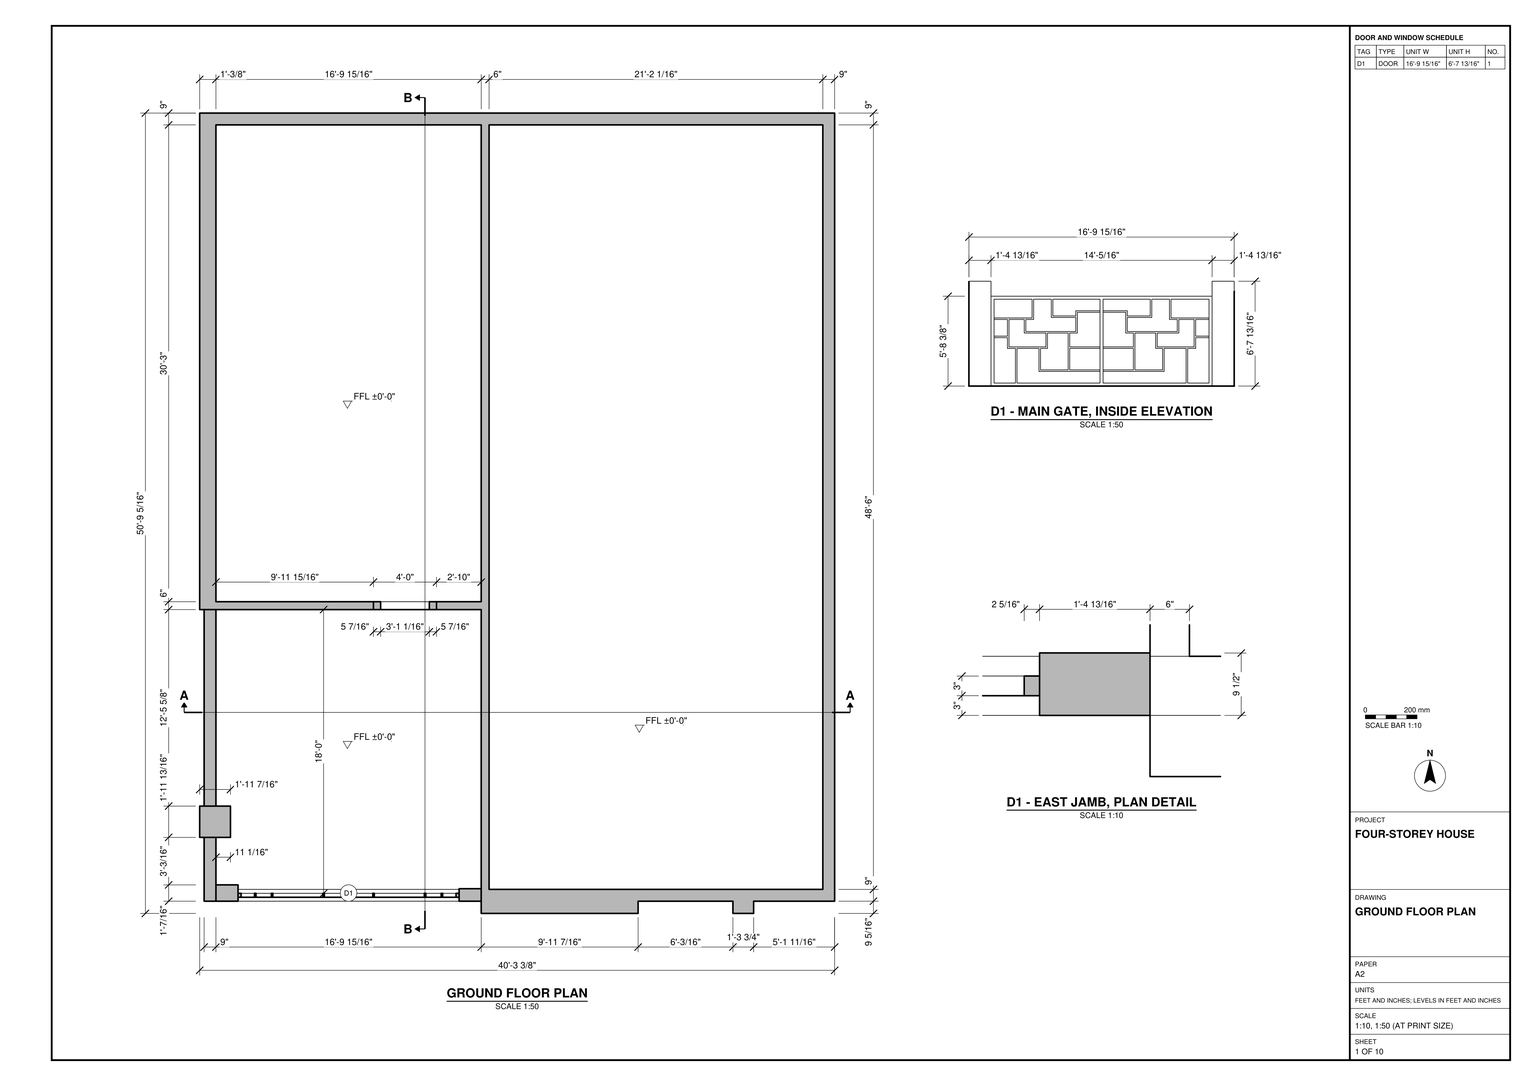
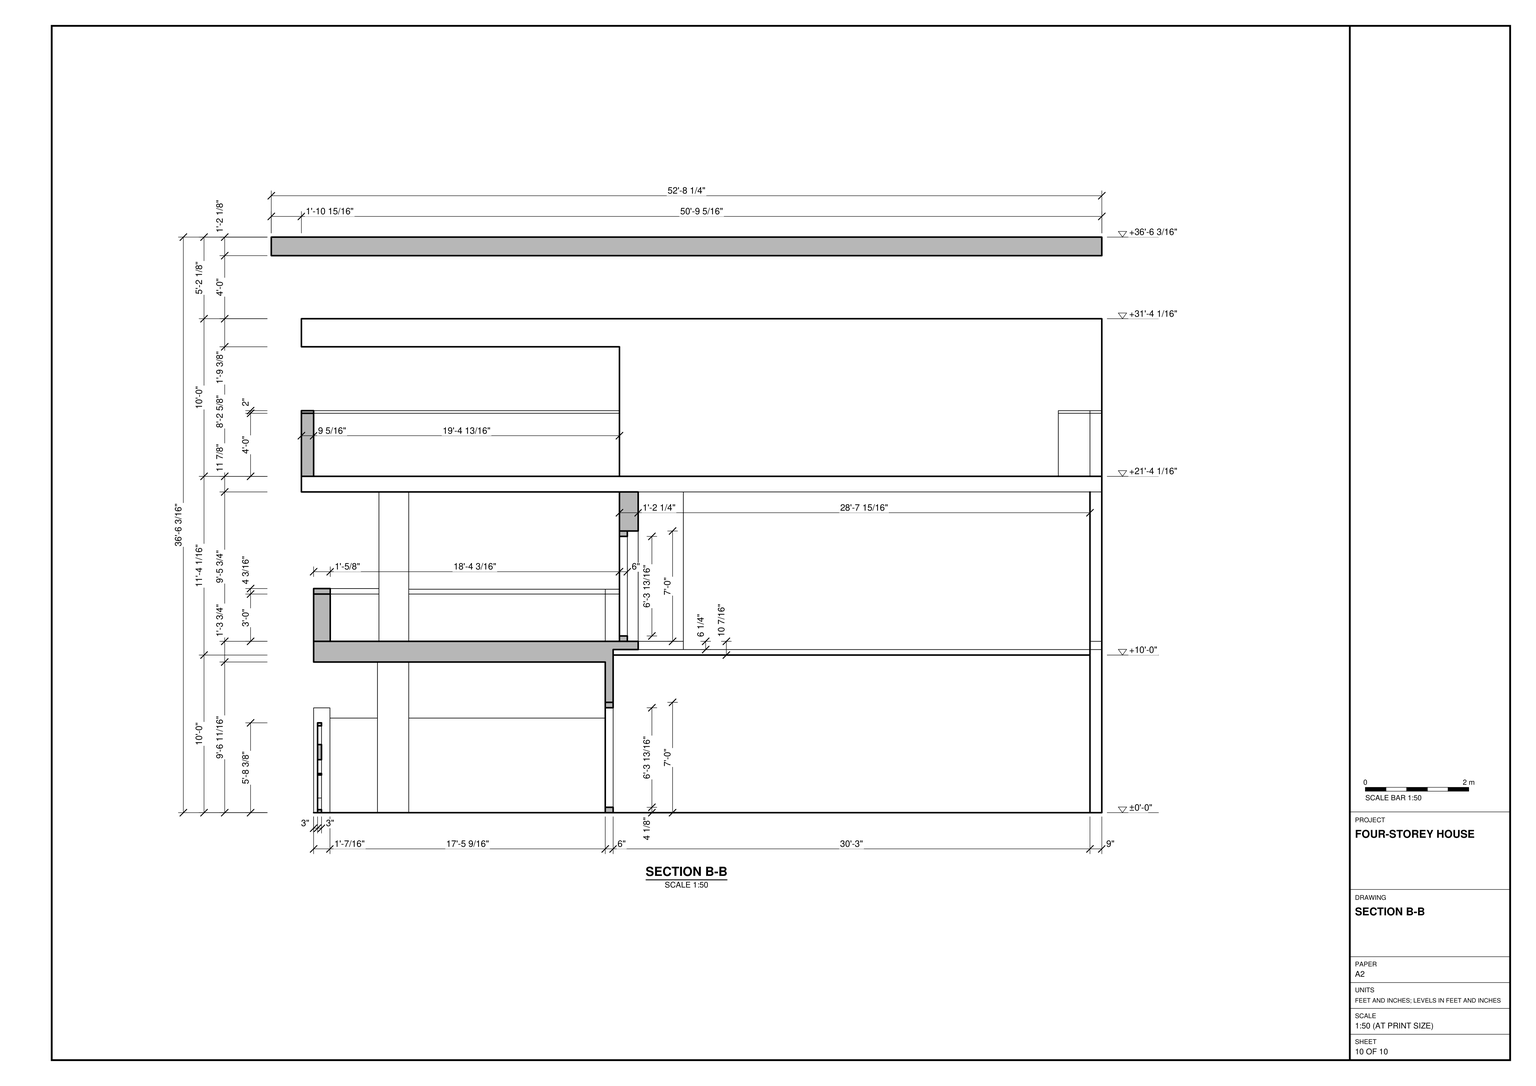
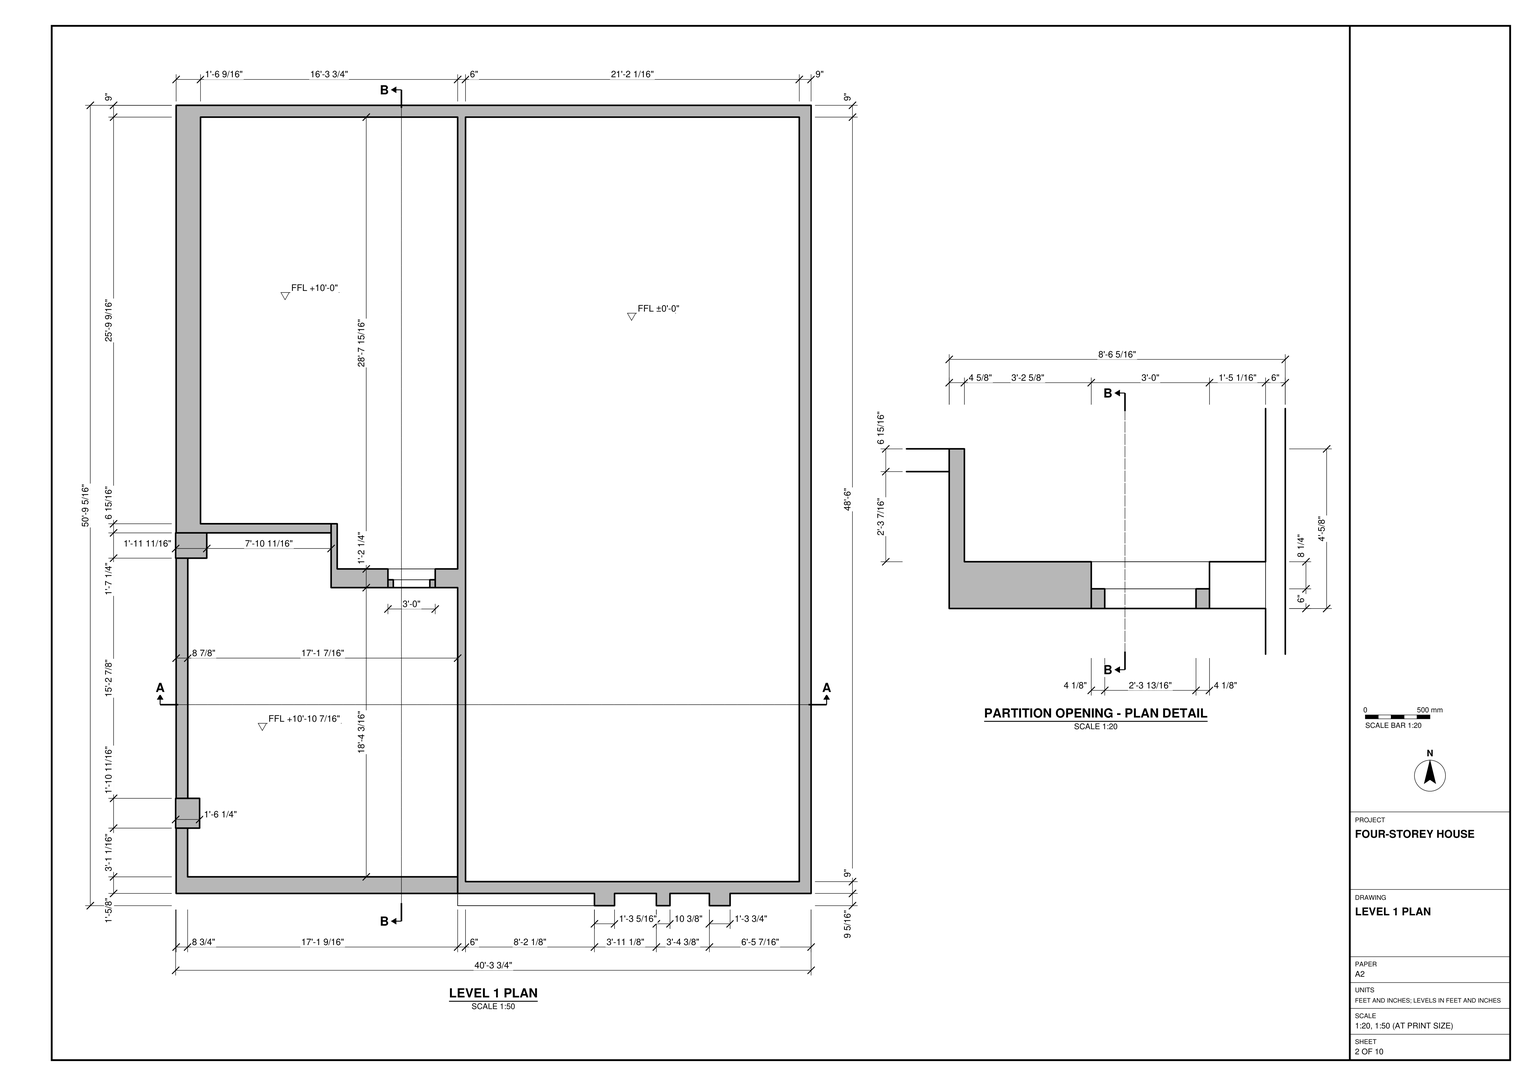
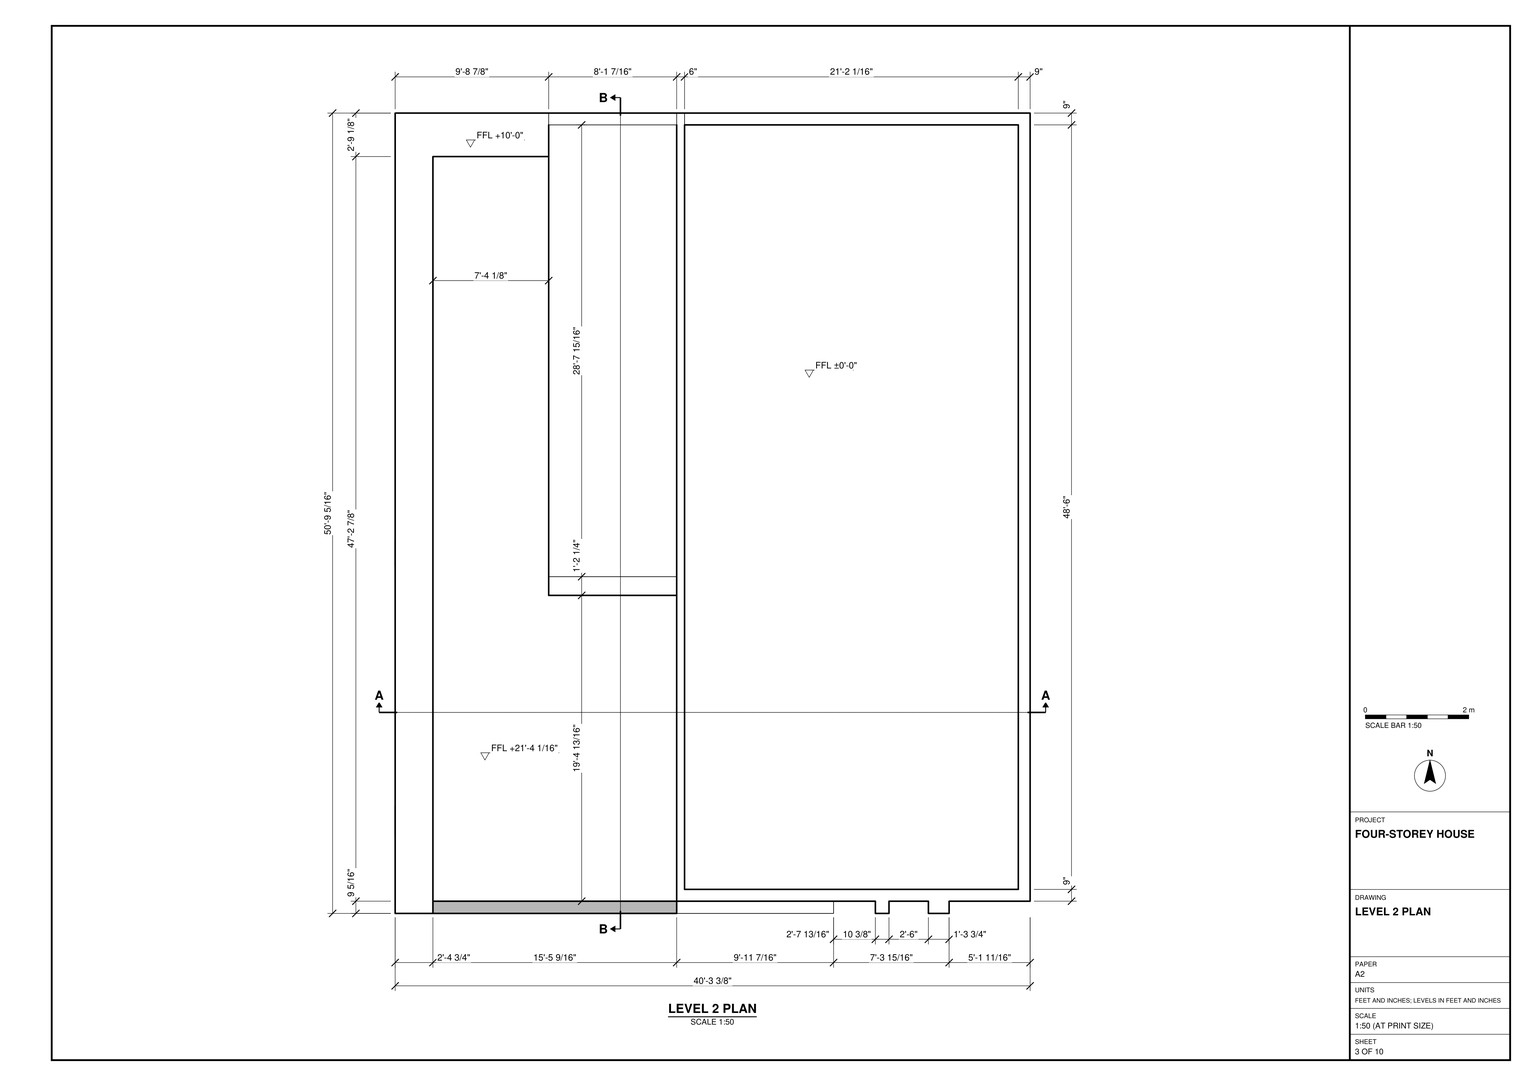
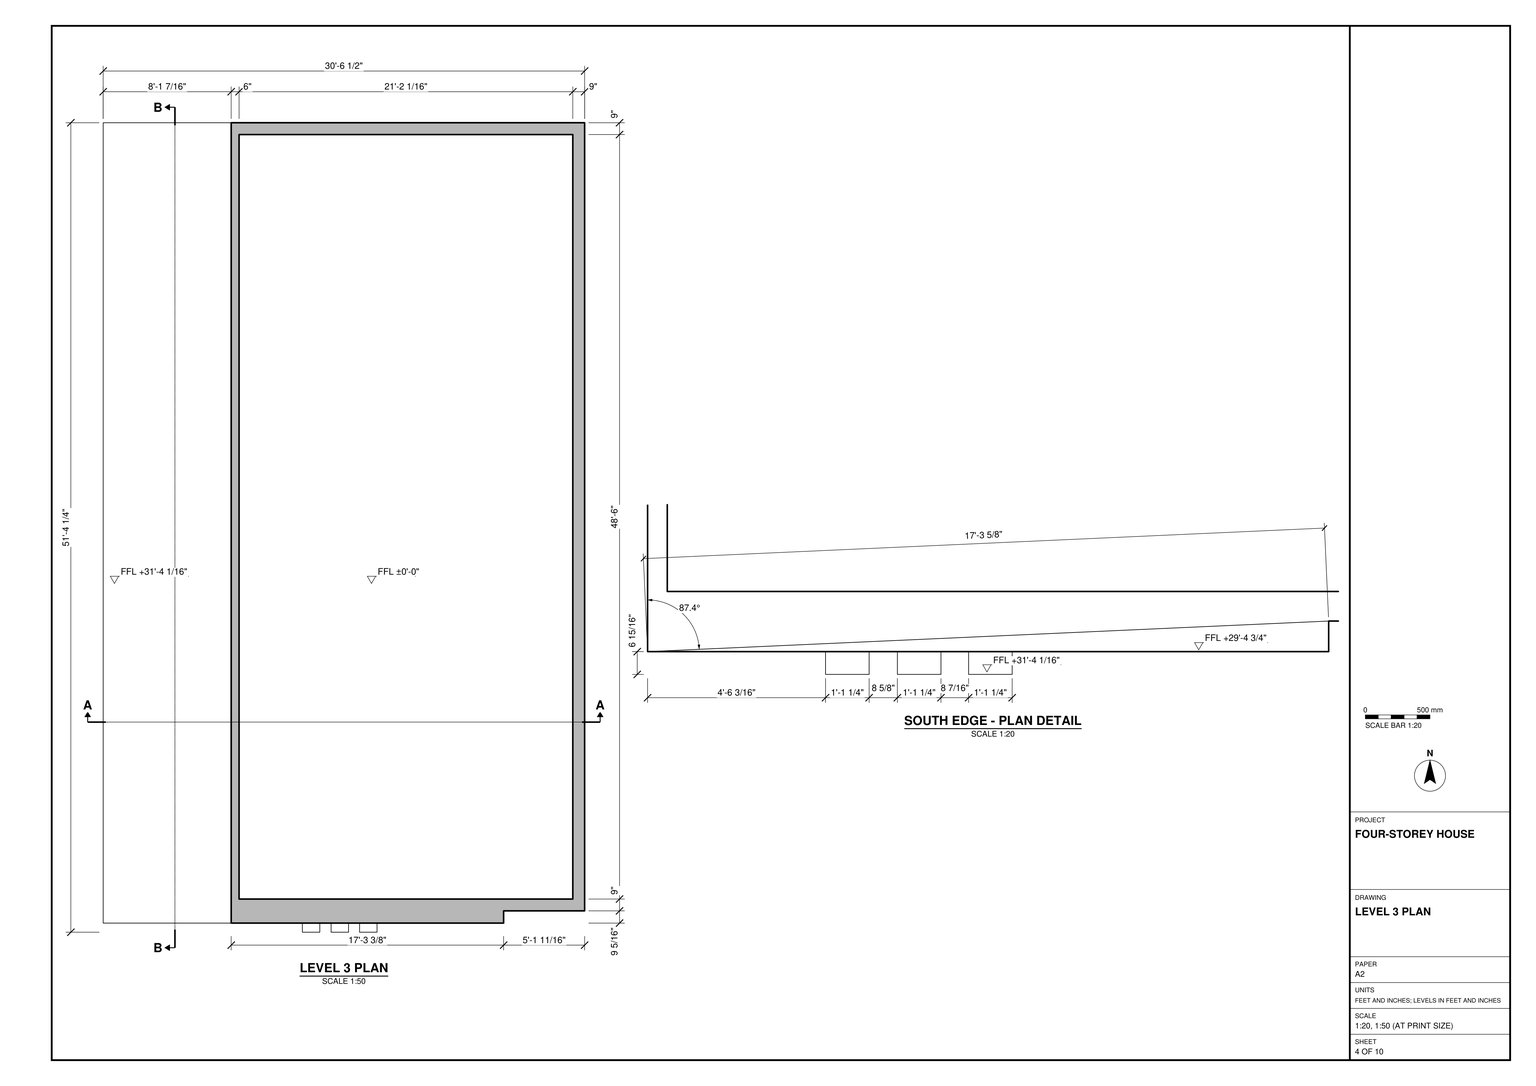
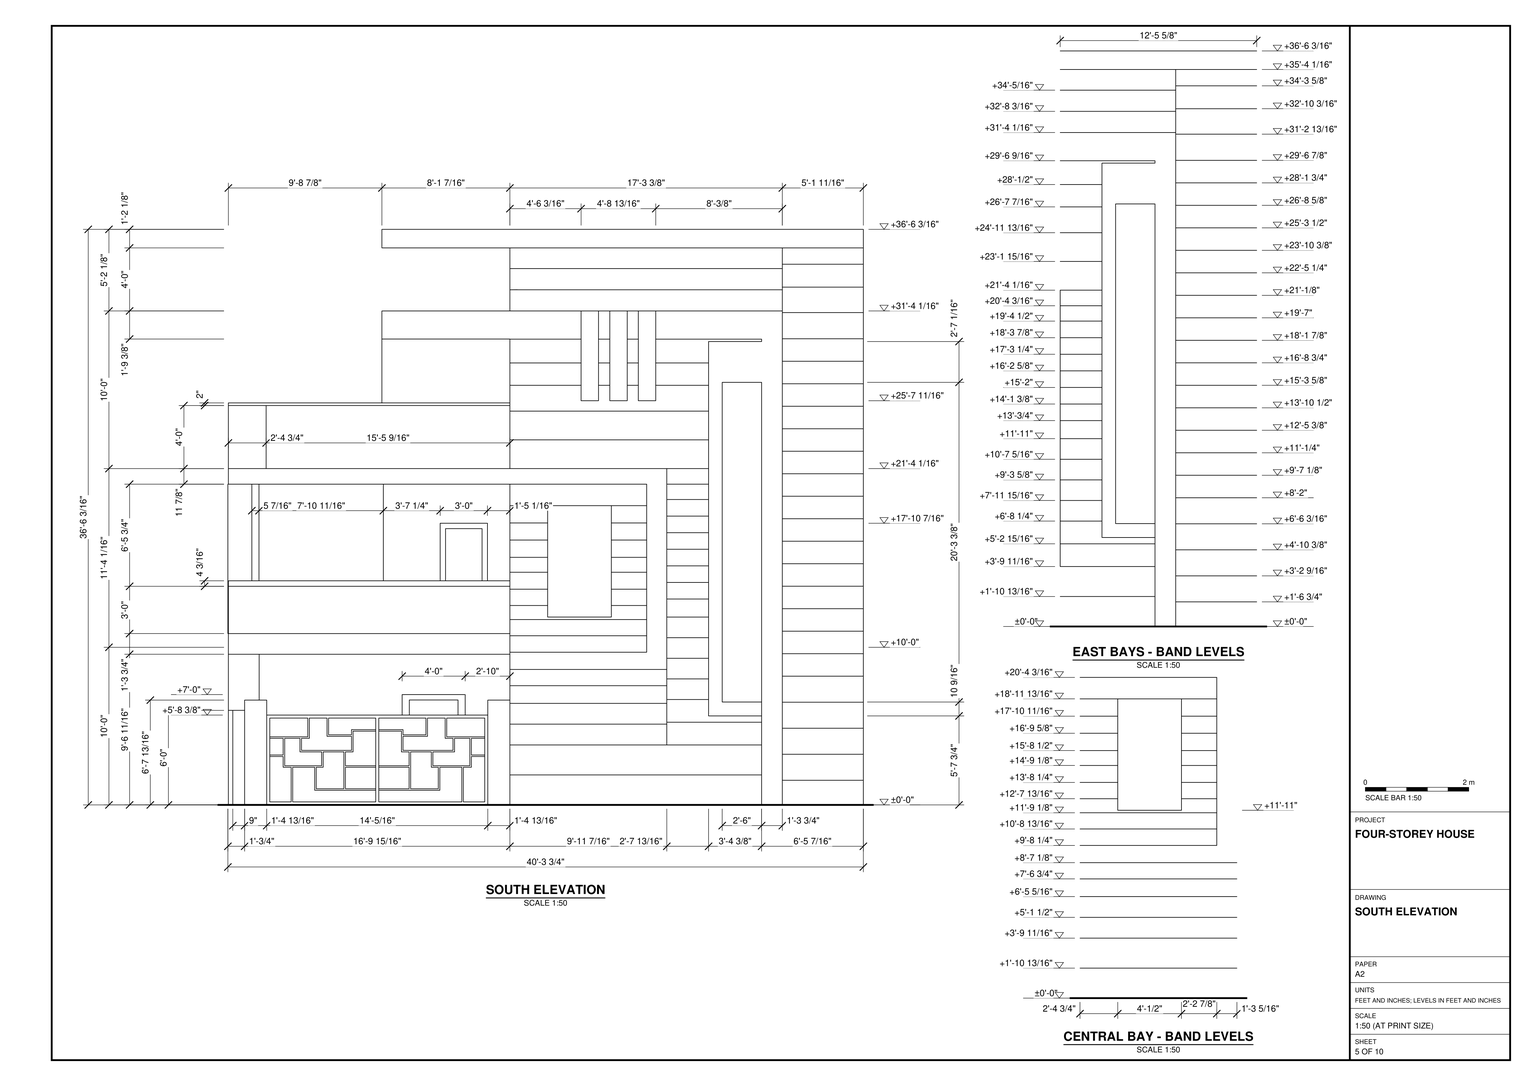
Build the four-storey house in SketchUp from task_files/diagram_01.pdf. Work in feet and inches. The overall width is 40'-3 3/4", the depth is 52'-8 1/4", and the height is 36'-6 3/16". Set the storey levels at ±0'-0", +10'-0", +21'-4 1/16" and +31'-4 1/16".

Use the ground floor plan to lay out the long right-hand bay and the narrower left-hand bay. Divide the left bay with a cross wall, leaving the opening near the lengthwise partition. At the front of the left bay, model the main gate between its posts, with the paired rectangular patterns shown in the gate elevation. Follow the dimensioned wall thicknesses, jambs and offsets rather than using one wall thickness throughout.

On the first upper level, follow the stepped partition and the change in floor height between the front and rear of the left bay. Use the sections to set the slab edges, terrace parapets and projecting flat roof. Include stairs, built-in joinery and main furniture only where shown. Any decor or loose items shown may be represented by suitable library components.

Keep walls, slabs, roof and each furniture or joinery piece in separate groups or components, and use components for repeated parts. Save one SketchUp model as output_files/four_storey_house_with_a_patterned_entrance_gate.skp.

# SketchUp Ruby script. Lengths in inches.
U = 1.inch
M = Sketchup.active_model
def pt(a) = Geom::Point3d.new(a.map { |v| v * U })
def face(e, loops, mat)
  f = e.add_face(loops[0].map { |a| pt(a) })
  loops[1..].each { |l| e.add_face(l.map { |a| pt(a) }).erase! }
  f.material = f.back_material = mat if mat
  f
end
# faces: each face lists its corners as indices into pts; further lists are holes
def faces(e, pts, list, mat = nil) = list.each { |f| face(e, (f[0].is_a?(Array) ? f : [f]).map { |l| l.map { |i| pts[i] } }, mat) }
# xy, xz, yz: faces in a plane at the given z, y or x. An outline is a flat list of corners, or four numbers for a rectangle; further outlines are holes
def ring(l) = l.size == 4 ? [[l[0], l[1]], [l[2], l[1]], [l[2], l[3]], [l[0], l[3]]] : l.each_slice(2).to_a
def flat(e, list, mat, &to3) = list.each { |f| face(e, (f[0].is_a?(Array) ? f : [f]).map { |l| ring(l).map { |u, v| to3.(u, v) } }, mat) }
def xy(e, z, list, mat = nil) = flat(e, list, mat) { |x, y| [x, y, z] }
def xz(e, y, list, mat = nil) = flat(e, list, mat) { |x, z| [x, y, z] }
def yz(e, x, list, mat = nil) = flat(e, list, mat) { |y, z| [x, y, z] }
def lines(e, pts, list) = list.each { |a, b| e.add_line(pt(pts[a]), pt(pts[b])) }
# prism: a flat outline (further loops are holes) pulled along v
def prism(e, loops, v, mat = nil)
  f = face(e, loops, mat); d = Geom::Vector3d.new(v.map { |x| x * U })
  f.pushpull(f.normal.samedirection?(d) ? d.length : -d.length)
end
def box(e, o, s, mat = nil) = prism(e, [[o, [o[0] + s[0], o[1], o[2]], [o[0] + s[0], o[1] + s[1], o[2]], [o[0], o[1] + s[1], o[2]]]], [0, 0, s[2]], mat)
def at(x, y, z, deg = 0) = Geom::Transformation.translation(pt([x, y, z])) * Geom::Transformation.rotation(ORIGIN, Z_AXIS, deg.degrees)
def axes(o, x, y, z) = Geom::Transformation.new([*x, 0, *y, 0, *z, 0, *pt(o).to_a, 1])
def part(name) = M.definitions.add(name)
# library, detail: a bought-in or finely detailed component or shape, given as its bounding box
def library(name, o, s) = part(name).tap { |d| box(d.entities, o, s) }
def detail(e, o, s) = box(e.add_group.entities, o, s)
def put(e, d, t, mat = nil) = e.add_instance(d, t).tap { |i| i.material = mat if mat }
def group(e, t, mat = nil) = e.add_group.tap { |g| g.transformation = t; g.material = mat if mat }.entities
root = M.entities
M.materials.add("[Cladding_Siding_Tan]").color = [99, 77, 58]
M.materials.add("[Color C08]").color = [102, 51, 0]
M.materials.add("[Color G02]").color = [153, 255, 153]
M.materials.add("[Color M00]").color = [255, 255, 255]
M.materials.add("[Color M04]").color = [142, 142, 142]
M.materials.add("[Terrazzo]").color = [241, 241, 241]
M.materials.add("[Translucent Glass Blue]").color = [100, 149, 237]
M.materials["[Translucent Glass Blue]"].alpha = 0.5
M.materials.add("[Translucent Glass Gray]").color = [128, 128, 128]
M.materials["[Translucent Glass Gray]"].alpha = 0.5
M.materials.add("[WarmGray8]").color = [97, 85, 76]
M.materials.add("[White]").color = [255, 255, 255]
M.materials.add("timber-panels-light").color = [206, 147, 85]
c1 = part("main gate")
g1 = group(c1.entities,at(83.99,9.51,0,-90),"[Cladding_Siding_Tan]")
xy(g1,0,[[-2.91,-83.99,9.51,-72],[0,48,9.51,59.99]])
xy(g1,84,[[-2.91,-83.99,9.51,-72],[0,48,9.51,59.99]],"[Cladding_Siding_Tan]")
xz(g1,-83.99,[[-2.91,0,9.51,84]])
xz(g1,-72,[[-2.91,0,9.51,84]])
xz(g1,48,[[0,0,9.51,84]])
xz(g1,59.99,[[0,0,9.51,84]])
yz(g1,-2.91,[[-83.99,0,-72,84]])
yz(g1,0,[[48,0,59.99,84]])
yz(g1,9.51,[[-83.99,0,-72,84],[48,0,59.99,84]],"[Cladding_Siding_Tan]")
g2 = group(g1,at(6.51,-72,0))
xy(g2,0,[[-3,0,0,120]],"[WarmGray8]")
xy(g2,2.4,[[-3,1.67,0,13.27],[-3,106.73,0,118.33]],"[WarmGray8]")
xy(g2,2.4,[[-3,14.1,0,59.17],[-3,60.83,0,105.9]],"[White]")
xy(g2,11.74,[[-3,26.04,0,59.17],[-3,60.83,0,93.96]],"[White]")
xy(g2,12.94,[[-3,26.87,0,41.88],[-3,78.12,0,93.13]],"[WarmGray8]")
xy(g2,12.94,[[-3,42.72,0,59.17],[-3,60.83,0,77.28]],"[White]")
xy(g2,30.19,[[-3,26.87,0,30.65],[-3,89.35,0,93.13]],"[WarmGray8]")
xy(g2,30.19,[[-3,8.92,0,13.27],[-3,14.1,0,26.04],[-3,42.72,0,59.17],[-3,60.83,0,77.28],[-3,93.96,0,105.9],
  [-3,106.73,0,111.08]],"[White]")
xy(g2,31.39,[[-3,9.76,0,29.8125],[-3,90.1875,0,110.24]],"[WarmGray8]")
xy(g2,31.39,[[-3,42.72,0,59.17],[-3,60.83,0,77.28]],"[White]")
xy(g2,38.8,[[-3,1.67,0,8.92],[-3,111.08,0,118.33]],"[White]")
xy(g2,40,[[-3,1.67,0,8.92],[-3,111.08,0,118.33]],"[White]")
xy(g2,42.49,[[-3,18.06,0,29.8125],[-3,30.65,0,41.88],[-3,78.12,0,89.35],[-3,90.1875,0,101.94]],"[WarmGray8]")
xy(g2,42.49,[[-3,42.72,0,46.86],[-3,73.14,0,77.28]],"[White]")
xy(g2,43.69,[[-3,18.89,0,46.03],[-3,73.97,0,101.11]],"[WarmGray8]")
xy(g2,53.37,[[-3,9.76,0,18.06],[-3,18.89,0,23.13],[-3,96.87,0,101.11],[-3,101.94,0,110.24]],"[WarmGray8]")
xy(g2,53.37,[[-3,1.67,0,8.92],[-3,111.08,0,118.33]],"[White]")
xy(g2,54.57,[[-3,1.67,0,22.3],[-3,97.7,0,118.33]],"[White]")
xy(g2,54.97,[[-3,32.74,0,46.03],[-3,73.97,0,87.26]],"[WarmGray8]")
xy(g2,56.17,[[-3,33.57,0,46.03],[-3,73.97,0,86.43]],"[White]")
xy(g2,59.14,[[-3,46.86,0,59.17],[-3,60.83,0,73.14]],"[White]")
xy(g2,60.34,[[-3,46.03,0,59.17],[-3,60.83,0,73.97]],"[White]")
xy(g2,69.6,[[-3,23.13,0,32.74],[-3,60.83,0,86.43],[-3,87.26,0,96.87]],"[WarmGray8]")
xy(g2,69.6,[[-3,1.67,0,22.3],[-3,33.57,0,59.17],[-3,97.7,0,118.33]],"[White]")
xy(g2,72,[[-3,0,0,120]],"[WarmGray8]")
xz(g2,0,[[-3,0,0,72]],"[WarmGray8]")
xz(g2,1.67,[[-3,38.8,0,40]],"[WarmGray8]")
xz(g2,1.67,[[-3,2.4,0,38.8],[-3,40,0,53.37],[-3,53.37,0,54.57],[-3,54.57,0,69.6]],"[White]")
xz(g2,8.92,[[-3,30.19,0,38.8],[-3,40,0,53.37]],"[White]")
xz(g2,9.76,[[-3,31.39,0,53.37]],"[WarmGray8]")
xz(g2,13.27,[[-3,2.4,0,30.19]],"[White]")
xz(g2,14.1,[[-3,2.4,0,30.19]],"[White]")
xz(g2,18.06,[[-3,42.49,0,53.37]],"[WarmGray8]")
xz(g2,18.89,[[-3,43.69,0,53.37]],"[WarmGray8]")
xz(g2,22.3,[[-3,54.57,0,69.6]],"[White]")
xz(g2,23.13,[[-3,53.37,0,69.6]],"[WarmGray8]")
xz(g2,26.04,[[-3,11.74,0,30.19]],"[White]")
xz(g2,26.87,[[-3,12.94,0,30.19]],"[WarmGray8]")
xz(g2,29.8125,[[-3,31.39,0,42.49]],"[WarmGray8]")
xz(g2,30.65,[[-3,30.19,0,42.49]],"[WarmGray8]")
xz(g2,32.74,[[-3,54.97,0,69.6]],"[WarmGray8]")
xz(g2,33.57,[[-3,56.17,0,69.6]],"[White]")
xz(g2,41.88,[[-3,12.94,0,42.49]],"[WarmGray8]")
xz(g2,42.72,[[-3,12.94,0,30.19],[-3,31.39,0,42.49]],"[White]")
xz(g2,46.03,[[-3,43.69,0,54.97]],"[WarmGray8]")
xz(g2,46.03,[[-3,56.17,0,60.34]],"[White]")
xz(g2,46.86,[[-3,42.49,0,59.14]],"[White]")
xz(g2,59.17,[[-3,59.14,0,60.34],[-3,60.34,0,69.6]],"[WarmGray8]")
xz(g2,59.17,[[-3,2.4,0,11.74],[-3,11.74,0,12.94],[-3,12.94,0,30.19],[-3,30.19,0,31.39],[-3,31.39,0,59.14]],"[White]")
xz(g2,60.83,[[-3,59.14,0,60.34]],"[WarmGray8]")
xz(g2,60.83,[[-3,2.4,0,11.74],[-3,11.74,0,12.94],[-3,12.94,0,30.19],[-3,30.19,0,31.39],[-3,31.39,0,59.14],
  [-3,60.34,0,69.6]],"[White]")
xz(g2,73.14,[[-3,42.49,0,59.14]],"[White]")
xz(g2,73.97,[[-3,43.69,0,54.97]],"[WarmGray8]")
xz(g2,73.97,[[-3,56.17,0,60.34]],"[White]")
xz(g2,77.28,[[-3,12.94,0,30.19],[-3,31.39,0,42.49]],"[White]")
xz(g2,78.12,[[-3,12.94,0,42.49]],"[WarmGray8]")
xz(g2,86.43,[[-3,56.17,0,69.6]],"[White]")
xz(g2,87.26,[[-3,54.97,0,69.6]],"[WarmGray8]")
xz(g2,89.35,[[-3,30.19,0,42.49]],"[WarmGray8]")
xz(g2,90.1875,[[-3,31.39,0,42.49]],"[WarmGray8]")
xz(g2,93.13,[[-3,12.94,0,30.19]],"[WarmGray8]")
xz(g2,93.96,[[-3,11.74,0,30.19]],"[White]")
xz(g2,96.87,[[-3,53.37,0,69.6]],"[WarmGray8]")
xz(g2,97.7,[[-3,54.57,0,69.6]],"[White]")
xz(g2,101.11,[[-3,43.69,0,53.37]],"[WarmGray8]")
xz(g2,101.94,[[-3,42.49,0,53.37]],"[WarmGray8]")
xz(g2,105.9,[[-3,2.4,0,30.19]],"[White]")
xz(g2,106.73,[[-3,2.4,0,30.19]],"[White]")
xz(g2,110.24,[[-3,31.39,0,53.37]],"[WarmGray8]")
xz(g2,111.08,[[-3,30.19,0,38.8],[-3,40,0,53.37]],"[White]")
xz(g2,118.33,[[-3,38.8,0,40]],"[WarmGray8]")
xz(g2,118.33,[[-3,2.4,0,38.8],[-3,40,0,53.37],[-3,53.37,0,54.57],[-3,54.57,0,69.6]],"[White]")
xz(g2,120,[[-3,0,0,72]],"[WarmGray8]")
yz(g2,-3,[[[0,0,120,72],[60.83,2.4,60.83,69.6,86.43,69.6,86.43,56.17,73.97,56.17,73.97,60.34,60.83,60.34,60.83,59.14,73.14,59.14,73.14,42.49,77.28,42.49,77.28,31.39,60.83,31.39,60.83,30.19,77.28,30.19,77.28,12.94,60.83,12.94,60.83,11.74,93.96,11.74,93.96,30.19,105.9,30.19,105.9,2.4],[14.1,2.4,14.1,30.19,26.04,30.19,26.04,11.74,59.17,11.74,59.17,12.94,42.72,12.94,42.72,30.19,59.17,30.19,59.17,31.39,42.72,31.39,42.72,42.49,46.86,42.49,46.86,59.14,59.17,59.14,59.17,60.34,46.03,60.34,46.03,56.17,33.57,56.17,33.57,69.6,59.17,69.6,59.17,2.4],[106.73,2.4,106.73,30.19,111.08,30.19,111.08,38.8,118.33,38.8,118.33,40,111.08,40,111.08,53.37,118.33,53.37,118.33,54.57,97.7,54.57,97.7,69.6,118.33,69.6,118.33,2.4],[1.67,2.4,1.67,69.6,22.3,69.6,22.3,54.57,1.67,54.57,1.67,53.37,8.92,53.37,8.92,40,1.67,40,1.67,38.8,8.92,38.8,8.92,30.19,13.27,30.19,13.27,2.4],[73.97,43.69,73.97,54.97,87.26,54.97,87.26,69.6,96.87,69.6,96.87,53.37,101.11,53.37,101.11,43.69],[18.89,43.69,18.89,53.37,23.13,53.37,23.13,69.6,32.74,69.6,32.74,54.97,46.03,54.97,46.03,43.69],[26.87,12.94,26.87,30.19,30.65,30.19,30.65,42.49,41.88,42.49,41.88,12.94],[78.12,12.94,78.12,42.49,89.35,42.49,89.35,30.19,93.13,30.19,93.13,12.94],[90.1875,31.39,90.1875,42.49,101.94,42.49,101.94,53.37,110.24,53.37,110.24,31.39],[9.76,31.39,9.76,53.37,18.06,53.37,18.06,42.49,29.8125,42.49,29.8125,31.39]]],"[WarmGray8]")
yz(g2,0,[[[0,0,120,72],[60.83,2.4,105.9,2.4,105.9,30.19,93.96,30.19,93.96,11.74,60.83,11.74,60.83,12.94,77.28,12.94,77.28,30.19,60.83,30.19,60.83,31.39,77.28,31.39,77.28,42.49,73.14,42.49,73.14,59.14,60.83,59.14,60.83,60.34,73.97,60.34,73.97,56.17,86.43,56.17,86.43,69.6,60.83,69.6],[14.1,2.4,59.17,2.4,59.17,69.6,33.57,69.6,33.57,56.17,46.03,56.17,46.03,60.34,59.17,60.34,59.17,59.14,46.86,59.14,46.86,42.49,42.72,42.49,42.72,31.39,59.17,31.39,59.17,30.19,42.72,30.19,42.72,12.94,59.17,12.94,59.17,11.74,26.04,11.74,26.04,30.19,14.1,30.19],[106.73,2.4,118.33,2.4,118.33,69.6,97.7,69.6,97.7,54.57,118.33,54.57,118.33,53.37,111.08,53.37,111.08,40,118.33,40,118.33,38.8,111.08,38.8,111.08,30.19,106.73,30.19],[1.67,2.4,13.27,2.4,13.27,30.19,8.92,30.19,8.92,38.8,1.67,38.8,1.67,40,8.92,40,8.92,53.37,1.67,53.37,1.67,54.57,22.3,54.57,22.3,69.6,1.67,69.6],[73.97,43.69,101.11,43.69,101.11,53.37,96.87,53.37,96.87,69.6,87.26,69.6,87.26,54.97,73.97,54.97],[18.89,43.69,46.03,43.69,46.03,54.97,32.74,54.97,32.74,69.6,23.13,69.6,23.13,53.37,18.89,53.37],[26.87,12.94,41.88,12.94,41.88,42.49,30.65,42.49,30.65,30.19,26.87,30.19],[78.12,12.94,93.13,12.94,93.13,30.19,89.35,30.19,89.35,42.49,78.12,42.49],[90.1875,31.39,110.24,31.39,110.24,53.37,101.94,53.37,101.94,42.49,90.1875,42.49],[9.76,31.39,29.8125,31.39,29.8125,42.49,18.06,42.49,18.06,53.37,9.76,53.37]]],"[WarmGray8]")
yz(g2,0,[[1.67,2.4,1.67,38.8,8.92,38.8,8.92,30.19,13.27,30.19,13.27,2.4],[14.1,2.4,14.1,30.19,26.04,30.19,26.04,11.74,59.17,11.74,59.17,2.4],[60.83,2.4,60.83,11.74,93.96,11.74,93.96,30.19,105.9,30.19,105.9,2.4],[106.73,2.4,106.73,30.19,111.08,30.19,111.08,38.8,118.33,38.8,118.33,2.4],[26.87,12.94,26.87,30.19,30.65,30.19,30.65,42.49,41.88,42.49,41.88,12.94],
  [42.72,12.94,59.17,30.19],[60.83,12.94,77.28,30.19],[78.12,12.94,78.12,42.49,89.35,42.49,89.35,30.19,93.13,30.19,93.13,12.94],[9.76,31.39,9.76,53.37,18.06,53.37,18.06,42.49,29.8125,42.49,29.8125,31.39],[42.72,31.39,42.72,42.49,46.86,42.49,46.86,59.14,59.17,59.14,59.17,31.39],
  [60.83,31.39,60.83,59.14,73.14,59.14,73.14,42.49,77.28,42.49,77.28,31.39],[90.1875,31.39,90.1875,42.49,101.94,42.49,101.94,53.37,110.24,53.37,110.24,31.39],[1.67,40,8.92,53.37],[111.08,40,118.33,53.37],[18.89,43.69,18.89,53.37,23.13,53.37,23.13,69.6,32.74,69.6,32.74,54.97,46.03,54.97,46.03,43.69],
  [73.97,43.69,73.97,54.97,87.26,54.97,87.26,69.6,96.87,69.6,96.87,53.37,101.11,53.37,101.11,43.69],[1.67,54.57,22.3,69.6],[97.7,54.57,118.33,69.6],[33.57,56.17,33.57,69.6,59.17,69.6,59.17,60.34,46.03,60.34,46.03,56.17],[73.97,56.17,73.97,60.34,60.83,60.34,60.83,69.6,86.43,69.6,86.43,56.17]],"timber-panels-light")
xy(root,0,[[406.3125,22.9375,406.3125,32.25,214.6875,32.25,214.6875,41.25,474.75,41.25,474.75,623.25,12.75,623.25,12.75,254.25,0.375,254.25,0.375,632.25,483.75,632.25,483.75,32.25,422.08,32.25,422.08,22.9375],[3.75,32.25,12.75,80.84],[12.75,32.25,214.6875,41.25],[12.75,41.25,214.6875,41.25,214.6875,254.25,180.66,254.25,180.66,260.25,132.66,260.25,132.66,254.25,12.75,254.25,12.75,104.65,23.8125,104.65,23.8125,80.84,12.75,80.84],[214.6875,41.25,214.6875,254.25,180.66,254.25,180.66,260.25,214.6875,260.25,214.6875,623.25,220.6875,623.25,220.6875,41.25],
  [220.6875,41.25,474.75,623.25],[0.375,80.84,3.75,104.65],[3.75,80.84,12.75,104.65],[12.75,80.84,23.8125,104.65],[3.75,104.65,12.75,254.25],
  [12.75,254.25,132.66,260.25],[12.75,260.25,214.6875,623.25]])
xy(root,45.67,[[214.6875,22.9375,334.125,32.25]])
xy(root,67.76,[[365.9375,22.9375,406.3125,32.25]])
xy(root,72,[[3.75,32.25,12.75,80.84],[3.75,104.65,12.75,254.25]],"[Color G02]")
xy(root,78.34,[[376.3125,22.9375,406.3125,32.25]])
xy(root,84,[[132.66,254.25,180.66,260.25]])
xy(root,114.6875,[[0.375,32.25,0.375,80.84,23.8125,80.84,23.8125,104.65,0.375,104.65,0.375,254.25,214.6875,254.25,214.6875,32.25]])
xy(root,116.25,[[214.6875,22.9375,318.8125,32.25]])
xy(root,120,[[12.75,260.25,214.6875,623.25]])
xy(root,124.1875,[[12.75,260.25,12.75,313.6875,118.35,313.6875,118.35,279.3125,214.6875,279.3125,214.6875,260.25],[12.75,313.6875,18.9375,623.25]])
xy(root,130.4375,[[0.375,32.25,0.375,81.97,9.125,81.97,9.125,44.89,214.6875,44.89,214.6875,32.25],[9.125,44.89,214.6875,44.89,214.6875,265.0625,197.61,265.0625,197.61,279.3125,161.61,279.3125,161.61,265.0625,118.35,265.0625,118.35,306.75,23.6875,306.75,23.6875,287.5,9.25,287.5,9.25,104.65,18.25,104.65,18.25,81.97,9.125,81.97],[0,81.97,0.375,104.65],[0.375,81.97,18.25,104.65],[0.375,104.65,9.25,287.5],
  [118.35,279.3125,122.98,313.6875],[0,287.5,0.375,306.75],[0.375,287.5,9.25,306.75],[9.25,287.5,23.6875,306.75]])
xy(root,166.4375,[[0.375,32.25,0.375,81.97,9.125,81.97,9.125,44.89,214.6875,44.89,214.6875,32.25],[0.375,104.65,9.25,287.5]])
xy(root,170.125,[[0.375,104.65,9.25,287.5]],"[Color M04]")
xy(root,170.625,[[0.375,32.25,214.6875,32.25,214.6875,44.89,9.125,44.89,9.125,81.97,0.375,81.97]],"[Color M04]")
xy(root,214.4375,[[161.61,265.0625,197.61,279.3125]])
xy(root,244.1875,[[214.6875,22.9375,221.1875,32.25],[221.1875,22.9375,318.8125,32.25],[0,81.97,0.375,104.65],[0.375,81.97,18.25,104.65],[118.35,265.0625,122.98,279.3125],
  [122.98,265.0625,214.6875,279.3125],[118.35,279.3125,122.98,306.75],[0,287.5,0.375,306.75],[0.375,287.5,23.6875,306.75],[0.375,306.75,118.35,313.6875],
  [118.35,306.75,122.98,313.6875]])
xy(root,244.1875,[[0.375,22.9375,0.375,81.97,18.25,81.97,18.25,104.65,0.375,104.65,0.375,287.5,23.6875,287.5,23.6875,306.75,118.35,306.75,118.35,265.0625,214.6875,265.0625,214.6875,22.9375]],"[Color M00]")
xy(root,256.0625,[[0.375,22.9375,0.375,632.25,117.25,632.25,117.25,599.15,29.125,599.15,29.125,22.9375],[29.125,22.9375,214.6875,32.25],[214.6875,22.9375,334.125,32.25],[29.125,32.25,214.6875,32.25,214.6875,265.0625,117.25,265.0625,117.25,599.15,29.125,599.15],[117.25,265.0625,214.6875,279.3125],
  [117.25,279.3125,214.6875,623.25],[117.25,623.25,214.6875,632.25]])
xy(root,304.0625,[[0.375,22.9375,29.125,32.25],[29.125,22.9375,214.6875,32.25],[0.375,32.25,0.375,632.25,117.25,632.25,117.25,599.15,29.125,599.15,29.125,32.25]])
xy(root,306.0625,[[0.375,22.9375,214.6875,32.25],[0.375,32.25,29.125,32.25,29.125,599.15,117.25,599.15,117.25,632.25,0.375,632.25]],"[Color M04]")
xy(root,307.71,[[268.875,16,282.15,22.9375],[290.75,16,304.02,22.9375],[312.4375,16,325.71,22.9375]],"[Color M04]")
xy(root,321.71,[[376.3125,22.9375,406.3125,32.25]])
xy(root,352.78,[[365.9375,22.9375,406.3125,32.25]])
xy(root,354.59,[[214.6875,22.9375,406.3125,32.25]])
xy(root,354.6875,[[117.25,22.9375,214.6875,265.0625]],"[Color M00]")
xy(root,376.0625,[[117.25,22.9375,214.6875,632.25]],"[Color G02]")
xy(root,376.0625,[[268.875,16,282.15,22.9375],[290.75,16,304.02,22.9375],[312.4375,16,325.71,22.9375]],"[Color M04]")
xy(root,424.0625,[[117.25,0,117.25,632.25,214.6875,632.25,214.6875,22.9375,422.08,22.9375,422.08,32.25,483.75,32.25,483.75,0],[214.6875,22.9375,214.6875,632.25,220.6875,632.25,220.6875,41.25,474.75,41.25,474.75,623.25,220.6875,623.25,220.6875,632.25,483.75,632.25,483.75,32.25,422.08,32.25,422.08,22.9375]])
xy(root,438.1875,[[117.25,0,483.75,632.25]],"[Color M00]")
xz(root,0,[[117.25,424.0625,483.75,438.1875]],"[Color M00]")
xz(root,16,[[268.875,307.71,282.15,376.0625],[290.75,307.71,304.02,376.0625],[312.4375,307.71,325.71,376.0625]],"[Color M04]")
xz(root,22.9375,[[406.3125,0,422.08,0,422.08,376.0625,325.71,376.0625,325.71,354.59,406.3125,354.59,406.3125,352.78,365.9375,352.78,365.9375,67.76,406.3125,67.76,406.3125,78.34,376.3125,78.34,376.3125,321.71,406.3125,321.71],[268.875,307.71,282.15,354.59],[290.75,307.71,304.02,354.59],[312.4375,307.71,325.71,354.59],[214.6875,354.59,268.875,354.59,268.875,376.0625,117.25,376.0625,117.25,354.6875,214.6875,354.6875],
  [268.875,354.59,282.15,376.0625],[282.15,354.59,290.75,376.0625],[290.75,354.59,304.02,376.0625],[304.02,354.59,312.4375,376.0625],[312.4375,354.59,325.71,376.0625]])
xz(root,22.9375,[[214.6875,45.67,334.125,61.49],[214.6875,61.49,334.125,77.3],[214.6875,77.3,334.125,90.77],[214.6875,90.77,334.125,103.13],[0.375,256.0625,29.125,304.0625],
  [214.6875,376.0625,422.08,392.1875],[214.6875,392.1875,422.08,408.3125],[214.6875,408.3125,422.08,424.0625]],"[Color G02]")
xz(root,22.9375,[[214.6875,103.13,334.125,103.13,334.125,256.0625,0.375,256.0625,0.375,244.1875,318.8125,244.1875,318.8125,116.25,214.6875,116.25]],"[Color M00]")
xz(root,22.9375,[[0.375,304.0625,214.6875,306.0625]],"[Color M04]")
xz(root,22.9375,[[29.125,256.0625,214.6875,304.0625]],"[Translucent Glass Blue]")
xz(root,32.25,[[0.375,114.6875,214.6875,130.4375]])
xz(root,32.25,[[3.75,0,12.75,72],[214.6875,0,406.3125,22.83],[422.08,0,483.75,18.75],[422.08,18.75,483.75,38.5625],[214.6875,22.83,406.3125,45.67],
  [422.08,38.5625,483.75,58.375],[334.125,45.67,406.3125,62.96],[422.08,58.375,483.75,78.1875],[334.125,62.96,406.3125,62.96,406.3125,67.76,365.9375,67.76,365.9375,80.25,334.125,80.25],[422.08,78.1875,483.75,98],
  [334.125,80.25,365.9375,95.94],[334.125,95.94,365.9375,111.62],[422.08,98,483.75,115.125],[334.125,111.62,365.9375,127.31],[422.08,115.125,483.75,132.25],
  [214.6875,116.25,318.8125,128.79],[334.125,127.31,365.9375,143],[214.6875,128.79,318.8125,141.125],[422.08,132.25,483.75,149.375],[214.6875,141.125,318.8125,141.125,318.8125,151.8125,291.93,151.8125,291.93,143.02,243.43,143.02,243.43,151.8125,214.6875,151.8125],
  [334.125,143,365.9375,156.75],[422.08,149.375,483.75,166.5],[214.6875,151.8125,243.43,164.22],[291.93,151.8125,318.8125,164.22],[334.125,156.75,365.9375,169.37],
  [214.6875,164.22,243.43,177.12],[291.93,164.22,318.8125,177.12],[422.08,166.5,483.75,183.625],[334.125,169.37,365.9375,182],[214.6875,177.12,243.43,188.48],
  [291.93,177.12,318.8125,188.48],[334.125,182,365.9375,194.62],[422.08,183.625,483.75,200.75],[214.6875,188.48,243.43,201.65],[291.93,188.48,318.8125,201.65],
  [334.125,194.62,365.9375,207.25],[422.08,200.75,483.75,217.875],[214.6875,201.65,243.43,214.66],[291.93,201.65,318.8125,214.66],[334.125,207.25,365.9375,219.87],
  [214.6875,214.66,243.43,227.83],[291.93,214.66,318.8125,227.83],[422.08,217.875,483.75,235],[334.125,219.87,365.9375,232.5],[214.6875,227.83,318.8125,244.1875],
  [334.125,232.5,365.9375,244.1875],[422.08,235,483.75,252.125],[334.125,244.1875,365.9375,256.0625],[422.08,252.125,483.75,269.25],[214.6875,256.0625,365.9375,277.93],
  [422.08,269.25,483.75,286.375],[214.6875,277.93,365.9375,299.79],[422.08,286.375,483.75,303.5],[214.6875,299.79,365.9375,319.45],[422.08,303.5,483.75,320.625],
  [214.6875,319.45,365.9375,336.48],[422.08,320.625,483.75,337.75],[214.6875,336.48,365.9375,336.48,365.9375,352.78,406.3125,352.78,406.3125,354.59,214.6875,354.59],[422.08,337.75,483.75,354.875],[422.08,354.875,483.75,374.8125],
  [422.08,374.8125,483.75,394.1875],[422.08,394.1875,483.75,411.625],[422.08,411.625,483.75,424.0625]],"[Color G02]")
xz(root,32.25,[[0.375,166.4375,214.6875,170.625],[29.125,304.0625,214.6875,306.0625]],"[Color M04]")
xz(root,32.25,[[243.43,143.02,291.93,227.83]],"[Terrazzo]")
xz(root,32.25,[[0.375,130.4375,214.6875,166.4375],[29.125,256.0625,214.6875,304.0625]],"[Translucent Glass Blue]")
xz(root,32.25,[[376.3125,78.34,406.3125,321.71]],"[Translucent Glass Gray]")
xz(root,41.25,[[220.6875,0,474.75,256.0625],[220.6875,256.0625,474.75,424.0625]])
xz(root,44.89,[[9.125,166.4375,214.6875,170.625]],"[Color M04]")
xz(root,44.89,[[9.125,130.4375,214.6875,166.4375]],"[Translucent Glass Blue]")
xz(root,80.84,[[3.75,0,12.75,72]])
xz(root,80.84,[[0.375,0,3.75,72],[12.75,0,23.8125,0,23.8125,114.6875,0.375,114.6875,0.375,72,12.75,72]],"[Color G02]")
xz(root,81.97,[[0.375,130.4375,9.125,166.4375],[0.375,166.4375,9.125,170.625]])
xz(root,81.97,[[0,130.4375,0.375,130.4375,0.375,170.625,9.125,170.625,9.125,130.4375,18.25,130.4375,18.25,244.1875,0,244.1875]],"[Color G02]")
xz(root,104.65,[[0.375,0,3.75,72],[3.75,0,12.75,72],[0.375,130.4375,9.25,166.4375],[0.375,166.4375,9.25,170.125]])
xz(root,104.65,[[12.75,0,12.75,72,0.375,72,0.375,114.6875,23.8125,114.6875,23.8125,0],[0,130.4375,0,244.1875,18.25,244.1875,18.25,130.4375,9.25,130.4375,9.25,170.125,0.375,170.125,0.375,130.4375]],"[Color G02]")
xz(root,254.25,[[3.75,0,12.75,72]])
xz(root,254.25,[[0.375,0,3.75,72],[12.75,0,132.66,0,132.66,84,180.66,84,180.66,0,214.6875,0,214.6875,114.6875,0.375,114.6875,0.375,72,12.75,72]],"[Color G02]")
xz(root,260.25,[[12.75,0,12.75,120,214.6875,120,214.6875,0,180.66,0,180.66,84,132.66,84,132.66,0],[12.75,120,214.6875,124.1875]])
xz(root,265.0625,[[118.35,130.4375,161.61,130.4375,161.61,214.4375,197.61,214.4375,197.61,130.4375,214.6875,130.4375,214.6875,244.1875,118.35,244.1875],[117.25,256.0625,214.6875,354.6875]],"[Color G02]")
xz(root,279.3125,[[[118.35,124.1875,118.35,130.4375,122.98,130.4375,122.98,244.1875,214.6875,244.1875,214.6875,124.1875],[161.61,130.4375,197.61,214.4375]]])
xz(root,287.5,[[0.375,130.4375,9.25,166.4375],[0.375,166.4375,9.25,170.125]])
xz(root,287.5,[[0,130.4375,0.375,130.4375,0.375,170.125,9.25,170.125,9.25,130.4375,23.6875,130.4375,23.6875,244.1875,0,244.1875]],"[Color G02]")
xz(root,306.75,[[0,130.4375,0.375,244.1875],[0.375,130.4375,23.6875,244.1875]])
xz(root,306.75,[[23.6875,130.4375,118.35,244.1875]],"[Color G02]")
xz(root,313.6875,[[18.9375,124.1875,118.35,244.1875],[118.35,130.4375,122.98,244.1875]])
xz(root,599.15,[[29.125,304.0625,117.25,306.0625]])
xz(root,599.15,[[29.125,256.0625,117.25,304.0625]],"[Color G02]")
xz(root,623.25,[[12.75,0,214.6875,120],[220.6875,0,474.75,256.0625],[12.75,120,29.125,124.1875],[29.125,120,214.6875,124.1875],[18.9375,124.1875,29.125,244.1875],
  [29.125,124.1875,214.6875,244.1875],[220.6875,256.0625,474.75,424.0625]])
xz(root,632.25,[[0.375,0,483.75,256.0625],[0.375,256.0625,0.375,304.0625,117.25,304.0625,117.25,376.0625,214.6875,376.0625,214.6875,424.0625,483.75,424.0625,483.75,256.0625]],"[Color G02]")
xz(root,632.25,[[117.25,424.0625,483.75,438.1875]],"[Color M00]")
xz(root,632.25,[[0.375,304.0625,117.25,306.0625]],"[Color M04]")
yz(root,0,[[81.97,130.4375,104.65,244.1875],[287.5,130.4375,306.75,244.1875]],"[Color G02]")
yz(root,0.375,[[80.84,0,80.84,114.6875,32.25,114.6875,32.25,130.4375,632.25,130.4375,632.25,0,254.25,0,254.25,114.6875,104.65,114.6875,104.65,0],[306.75,130.4375,632.25,244.1875],[22.9375,244.1875,632.25,256.0625],[22.9375,256.0625,632.25,304.0625]],"[Color G02]")
yz(root,0.375,[[32.25,166.4375,81.97,170.625],[104.65,166.4375,287.5,170.125],[22.9375,304.0625,632.25,306.0625]],"[Color M04]")
yz(root,0.375,[[32.25,130.4375,81.97,166.4375],[104.65,130.4375,287.5,166.4375]],"[Translucent Glass Blue]")
yz(root,3.75,[[32.25,0,80.84,72],[104.65,0,254.25,72]],"[Color G02]")
yz(root,9.125,[[44.89,166.4375,81.97,170.625]],"[Color M04]")
yz(root,9.125,[[44.89,130.4375,81.97,166.4375]],"[Translucent Glass Blue]")
yz(root,9.25,[[104.65,166.4375,254.25,170.125],[254.25,166.4375,287.5,170.125]],"[Color M04]")
yz(root,9.25,[[104.65,130.4375,254.25,166.4375],[254.25,130.4375,287.5,166.4375]],"[Translucent Glass Blue]")
yz(root,12.75,[[260.25,0,623.25,120],[260.25,120,623.25,124.1875]])
yz(root,12.75,[[32.25,0,41.25,72],[41.25,0,80.84,72],[104.65,0,254.25,72]],"[Color G02]")
yz(root,18.25,[[81.97,130.4375,104.65,244.1875]],"[Color G02]")
yz(root,18.9375,[[313.6875,124.1875,623.25,244.1875]])
yz(root,23.6875,[[287.5,130.4375,306.75,244.1875]],"[Color G02]")
yz(root,23.8125,[[80.84,0,104.65,114.6875]],"[Color G02]")
yz(root,29.125,[[22.9375,256.0625,32.25,304.0625],[32.25,304.0625,599.15,306.0625]])
yz(root,29.125,[[32.25,256.0625,599.15,304.0625]],"[Color G02]")
yz(root,117.25,[[599.15,256.0625,623.25,304.0625],[599.15,304.0625,623.25,306.0625],[623.25,304.0625,632.25,306.0625]])
yz(root,117.25,[[265.0625,256.0625,265.0625,354.6875,22.9375,354.6875,22.9375,376.0625,632.25,376.0625,632.25,306.0625,599.15,306.0625,599.15,256.0625]],"[Color G02]")
yz(root,117.25,[[0,424.0625,632.25,438.1875]],"[Color M00]")
yz(root,118.35,[[279.3125,124.1875,313.6875,130.4375],[306.75,130.4375,313.6875,244.1875]])
yz(root,118.35,[[265.0625,130.4375,306.75,244.1875]],"[Color G02]")
yz(root,122.98,[[279.3125,130.4375,313.6875,244.1875]])
yz(root,132.66,[[254.25,0,260.25,84]])
yz(root,161.61,[[265.0625,130.4375,279.3125,214.4375]])
yz(root,180.66,[[254.25,0,260.25,84]])
yz(root,197.61,[[265.0625,130.4375,279.3125,214.4375]],"[Color G02]")
yz(root,214.6875,[[260.25,0,623.25,120],[22.9375,114.6875,32.25,116.25],[260.25,120,623.25,124.1875],[279.3125,124.1875,623.25,256.0625],[32.25,130.4375,44.89,166.4375],
  [32.25,166.4375,44.89,170.625],[41.25,244.1875,265.0625,256.0625],[265.0625,244.1875,279.3125,256.0625],[22.9375,256.0625,32.25,304.0625],[265.0625,256.0625,279.3125,376.0625],
  [279.3125,256.0625,623.25,376.0625],[22.9375,304.0625,32.25,306.0625],[32.25,354.6875,41.25,376.0625],[41.25,354.6875,265.0625,376.0625]])
yz(root,214.6875,[[32.25,0,32.25,45.67,22.9375,45.67,22.9375,114.6875,254.25,114.6875,254.25,0],[44.89,130.4375,44.89,170.625,32.25,170.625,32.25,244.1875,265.0625,244.1875,265.0625,130.4375],[32.25,256.0625,32.25,354.59,22.9375,354.59,22.9375,354.6875,41.25,354.6875,41.25,256.0625],[41.25,256.0625,265.0625,354.6875],[22.9375,376.0625,632.25,424.0625]],"[Color G02]")
yz(root,220.6875,[[41.25,0,623.25,120],[41.25,120,623.25,256.0625],[41.25,256.0625,623.25,424.0625]])
yz(root,268.875,[[16,307.71,22.9375,376.0625]],"[Color M04]")
yz(root,282.15,[[16,307.71,22.9375,376.0625]],"[Color M04]")
yz(root,290.75,[[16,307.71,22.9375,376.0625]],"[Color M04]")
yz(root,304.02,[[16,307.71,22.9375,376.0625]],"[Color M04]")
yz(root,312.4375,[[16,307.71,22.9375,376.0625]],"[Color M04]")
yz(root,318.8125,[[22.9375,116.25,32.25,244.1875]])
yz(root,325.71,[[16,307.71,22.9375,376.0625]],"[Color M04]")
yz(root,334.125,[[22.9375,45.67,32.25,256.0625]])
yz(root,365.9375,[[22.9375,67.76,32.25,352.78]])
yz(root,376.3125,[[22.9375,78.34,32.25,321.71]])
yz(root,406.3125,[[22.9375,0,32.25,67.76],[22.9375,67.76,32.25,78.34],[22.9375,78.34,32.25,321.71],[22.9375,352.78,32.25,354.59]])
yz(root,422.08,[[22.9375,0,32.25,424.0625]])
yz(root,474.75,[[41.25,0,623.25,256.0625],[41.25,256.0625,623.25,424.0625]])
yz(root,483.75,[[32.25,0,632.25,424.0625]],"[Color G02]")
yz(root,483.75,[[0,424.0625,632.25,438.1875]],"[Color M00]")
p = [[9.25,254.25,124.1875],[214.6875,254.25,124.1875],[9.25,632.25,124.1875],[9.25,254.25,130.4375],[29.125,623.25,244.1875],[29.125,632.25,244.1875],
  [214.6875,623.25,244.1875],[214.6875,632.25,244.1875],[18.9375,623.25,244.1875],[18.9375,632.25,244.1875],[220.6875,41.25,120],[220.6875,32.25,120],
  [220.6875,623.25,256.0625],[220.6875,632.25,256.0625],[220.6875,41.25,424.0625],[220.6875,41.25,438.1875],[474.75,41.25,424.0625],[474.75,41.25,438.1875],
  [474.75,623.25,424.0625],[474.75,623.25,438.1875],[220.6875,632.25,436.0625],[220.6875,632.25,438.1875],[214.6875,22.9375,392.1875],[422.08,32.25,394.1875],
  [220.6875,623.25,376.0625],[220.6875,632.25,376.0625]]
lines(root,p,[[0,1],[0,2],[0,3],[4,5],[6,7],[8,9],[10,11],[12,13],[14,15],[16,17],[18,19],[20,21],
  [22,23],[24,25]])
put(root,c1,axes([12.75,32.25,0],[1.40248,0,0],[0,1,0],[0,0,0.95]))
g3 = group(root,at(132.66,254.25,0))
xy(g3,0,[[0,0,48,6]],"[Color C08]")
xy(g3,4.1,[[5.47,0,42.53,6]],"[Color C08]")
xy(g3,79.9,[[5.47,0,42.53,6]])
xy(g3,84,[[0,0,48,6]],"[Color C08]")
xz(g3,0,[[[0,0,48,84],[5.47,4.1,42.53,79.9]]],"[Color C08]")
xz(g3,0,[[5.47,4.1,42.53,79.9]],"[Translucent Glass Gray]")
xz(g3,6,[[[0,0,48,84],[5.47,4.1,42.53,79.9]]],"[Color C08]")
yz(g3,0,[[0,0,6,84]],"[Color C08]")
yz(g3,5.47,[[0,4.1,6,79.9]],"[Color C08]")
yz(g3,42.53,[[0,4.1,6,79.9]],"[Color C08]")
yz(g3,48,[[0,0,6,84]],"[Color C08]")
g4 = group(root,at(161.61,265.0625,130.4375))
xy(g4,0,[[0,0,36,6]],"[Color C08]")
xy(g4,4.1,[[4.1,0,31.9,6]],"[Color C08]")
xy(g4,79.9,[[4.1,0,31.9,6]])
xy(g4,84,[[0,0,36,6]],"[Color C08]")
xz(g4,0,[[[0,0,36,84],[4.1,4.1,31.9,79.9]]],"[Color C08]")
xz(g4,0,[[4.1,4.1,31.9,79.9]],"[Translucent Glass Gray]")
xz(g4,6,[[[0,0,36,84],[4.1,4.1,31.9,79.9]]],"[Color C08]")
yz(g4,0,[[0,0,6,84]],"[Color C08]")
yz(g4,4.1,[[0,4.1,6,79.9]],"[Color C08]")
yz(g4,31.9,[[0,4.1,6,79.9]],"[Color C08]")
yz(g4,36,[[0,0,6,84]],"[Color C08]")
